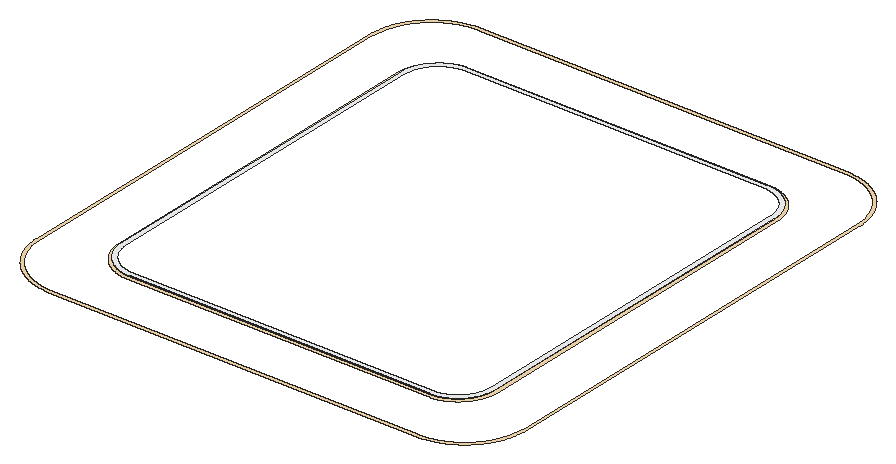
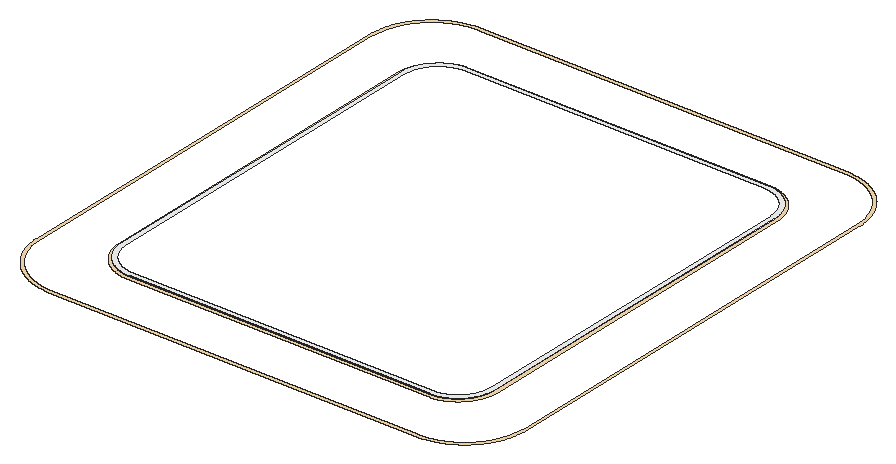
# SketchUp Ruby script. Lengths in inches.
U = 1.inch
M = Sketchup.active_model
def pt(a) = Geom::Point3d.new(a.map { |v| v * U })
def face(e, loops, mat)
  f = e.add_face(loops[0].map { |a| pt(a) })
  loops[1..].each { |l| e.add_face(l.map { |a| pt(a) }).erase! }
  f.material = f.back_material = mat if mat
  f
end
# faces: each face lists its corners as indices into pts; further lists are holes
def faces(e, pts, list, mat = nil) = list.each { |f| face(e, (f[0].is_a?(Array) ? f : [f]).map { |l| l.map { |i| pts[i] } }, mat) }
# xy, xz, yz: faces in a plane at the given z, y or x. An outline is a flat list of corners, or four numbers for a rectangle; further outlines are holes
def ring(l) = l.size == 4 ? [[l[0], l[1]], [l[2], l[1]], [l[2], l[3]], [l[0], l[3]]] : l.each_slice(2).to_a
def flat(e, list, mat, &to3) = list.each { |f| face(e, (f[0].is_a?(Array) ? f : [f]).map { |l| ring(l).map { |u, v| to3.(u, v) } }, mat) }
def xy(e, z, list, mat = nil) = flat(e, list, mat) { |x, y| [x, y, z] }
def xz(e, y, list, mat = nil) = flat(e, list, mat) { |x, z| [x, y, z] }
def yz(e, x, list, mat = nil) = flat(e, list, mat) { |y, z| [x, y, z] }
def lines(e, pts, list) = list.each { |a, b| e.add_line(pt(pts[a]), pt(pts[b])) }
# prism: a flat outline (further loops are holes) pulled along v
def prism(e, loops, v, mat = nil)
  f = face(e, loops, mat); d = Geom::Vector3d.new(v.map { |x| x * U })
  f.pushpull(f.normal.samedirection?(d) ? d.length : -d.length)
end
def box(e, o, s, mat = nil) = prism(e, [[o, [o[0] + s[0], o[1], o[2]], [o[0] + s[0], o[1] + s[1], o[2]], [o[0], o[1] + s[1], o[2]]]], [0, 0, s[2]], mat)
def at(x, y, z, deg = 0) = Geom::Transformation.translation(pt([x, y, z])) * Geom::Transformation.rotation(ORIGIN, Z_AXIS, deg.degrees)
def axes(o, x, y, z) = Geom::Transformation.new([*x, 0, *y, 0, *z, 0, *pt(o).to_a, 1])
def part(name) = M.definitions.add(name)
# library, detail: a bought-in or finely detailed component or shape, given as its bounding box
def library(name, o, s) = part(name).tap { |d| box(d.entities, o, s) }
def detail(e, o, s) = box(e.add_group.entities, o, s)
def put(e, d, t, mat = nil) = e.add_instance(d, t).tap { |i| i.material = mat if mat }
def group(e, t, mat = nil) = e.add_group.tap { |g| g.transformation = t; g.material = mat if mat }.entities
root = M.entities
M.materials.add("False Ceiling Light").color = [254, 223, 179]
M.materials.add("[Quartz Light Grey]").color = [251, 251, 252]
xy(root,115.32,[[[44.53,43.5,44.29,43.51,44.06,43.52,43.82,43.53,43.59,43.54,43.35,43.56,43.12,43.58,42.88,43.6,42.65,43.625,42.41,43.65,41.95,43.71,41.71,43.74,41.02,43.86,40.78,43.9,40.55,43.94,39.86,44.09,39.4,44.21,39.18,44.27,38.72,44.39,38.5,44.46,38.27,44.53,38.05,44.6,37.82,44.68,37.6,44.75,37.16,44.91,36.9375,44.99,36.72,45.08,36.28,45.26,36.0625,45.35,35.85,45.45,35.63,45.54,35.21,45.74,35,45.85,34.79,45.95,34.16,46.28,33.95,46.4,33.75,46.51,33.55,46.63,33.34,46.75,33.14,46.88,32.94,47,32.75,47.13,32.35,47.39,32.16,47.52,31.97,47.66,31.77,47.8,31.58,47.9375,31.4,48.08,31.21,48.22,31.02,48.37,30.84,48.51,30.48,48.81,30.3,48.97,30.12,49.12,29.94,49.28,29.77,49.4375,29.6,49.6,29.26,49.92,28.92,50.26,28.6,50.6,28.4375,50.77,28.28,50.94,28.12,51.12,27.97,51.3,27.81,51.48,27.51,51.84,27.37,52.02,27.22,52.21,27.08,52.4,26.9375,52.58,26.8,52.77,26.66,52.97,26.52,53.16,26.39,53.35,26.13,53.75,26,53.94,25.88,54.14,25.75,54.34,25.63,54.55,25.51,54.75,25.4,54.95,25.28,55.16,24.95,55.79,24.85,56,24.74,56.21,24.54,56.63,24.45,56.85,24.35,57.0625,24.26,57.28,24.08,57.72,23.99,57.9375,23.91,58.16,23.75,58.6,23.68,58.82,23.6,59.05,23.53,59.27,23.46,59.5,23.39,59.72,23.27,60.18,23.21,60.4,23.09,60.86,22.94,61.55,22.9,61.78,22.86,62.02,22.74,62.71,22.71,62.95,22.65,63.41,22.625,63.65,22.6,63.88,22.58,64.12,22.56,64.35,22.54,64.59,22.53,64.82,22.52,65.06,22.51,65.29,22.5,65.53,22.5,216.47,22.51,216.71,22.52,216.94,22.53,217.18,22.54,217.41,22.56,217.65,22.58,217.88,22.6,218.12,22.625,218.35,22.65,218.59,22.71,219.05,22.74,219.29,22.86,219.98,22.9,220.22,22.94,220.45,23.09,221.14,23.21,221.6,23.27,221.82,23.39,222.28,23.46,222.5,23.53,222.73,23.6,222.95,23.68,223.18,23.75,223.4,23.91,223.84,23.99,224.0625,24.08,224.28,24.26,224.72,24.35,224.9375,24.45,225.15,24.54,225.37,24.74,225.79,24.85,226,24.95,226.21,25.28,226.84,25.4,227.05,25.51,227.25,25.63,227.45,25.75,227.66,25.88,227.86,26,228.06,26.13,228.25,26.39,228.65,26.52,228.84,26.66,229.03,26.8,229.23,26.9375,229.42,27.08,229.6,27.22,229.79,27.37,229.98,27.51,230.16,27.81,230.52,27.97,230.7,28.12,230.88,28.28,231.06,28.4375,231.23,28.6,231.4,28.92,231.74,29.26,232.08,29.6,232.4,29.77,232.5625,29.94,232.72,30.12,232.88,30.3,233.03,30.48,233.19,30.84,233.49,31.02,233.63,31.21,233.78,31.4,233.92,31.58,234.0625,31.77,234.2,31.97,234.34,32.16,234.48,32.35,234.61,32.75,234.87,32.94,235,33.14,235.12,33.34,235.25,33.55,235.37,33.75,235.49,33.95,235.6,34.16,235.72,34.79,236.05,35,236.15,35.21,236.26,35.63,236.46,35.85,236.55,36.0625,236.65,36.28,236.74,36.72,236.92,36.9375,237.01,37.16,237.09,37.6,237.25,37.82,237.32,38.05,237.4,38.27,237.47,38.5,237.54,38.72,237.61,39.18,237.73,39.4,237.79,39.86,237.91,40.55,238.06,40.78,238.1,41.02,238.14,41.71,238.26,41.95,238.29,42.41,238.35,42.65,238.375,42.88,238.4,43.12,238.42,43.35,238.44,43.59,238.46,43.82,238.47,44.06,238.48,44.29,238.49,44.53,238.5,177.47,238.5,177.71,238.49,177.94,238.48,178.18,238.47,178.41,238.46,178.65,238.44,178.88,238.42,179.12,238.4,179.35,238.375,179.59,238.35,180.05,238.29,180.29,238.26,180.98,238.14,181.22,238.1,181.45,238.06,182.14,237.91,182.6,237.79,182.82,237.73,183.28,237.61,183.5,237.54,183.73,237.47,183.95,237.4,184.18,237.32,184.4,237.25,184.84,237.09,185.0625,237.01,185.28,236.92,185.72,236.74,185.9375,236.65,186.15,236.55,186.37,236.46,186.79,236.26,187,236.15,187.21,236.05,187.84,235.72,188.05,235.6,188.25,235.49,188.45,235.37,188.66,235.25,188.86,235.12,189.06,235,189.25,234.87,189.65,234.61,189.84,234.48,190.03,234.34,190.23,234.2,190.42,234.0625,190.6,233.92,190.79,233.78,190.98,233.63,191.16,233.49,191.52,233.19,191.7,233.03,191.88,232.88,192.06,232.72,192.23,232.5625,192.4,232.4,192.74,232.08,193.08,231.74,193.4,231.4,193.5625,231.23,193.72,231.06,193.88,230.88,194.03,230.7,194.19,230.52,194.49,230.16,194.63,229.98,194.78,229.79,194.92,229.6,195.0625,229.42,195.2,229.23,195.34,229.03,195.48,228.84,195.61,228.65,195.87,228.25,196,228.06,196.12,227.86,196.25,227.66,196.37,227.45,196.49,227.25,196.6,227.05,196.72,226.84,197.05,226.21,197.15,226,197.26,225.79,197.46,225.37,197.55,225.15,197.65,224.9375,197.74,224.72,197.92,224.28,198.01,224.0625,198.09,223.84,198.25,223.4,198.32,223.18,198.4,222.95,198.47,222.73,198.54,222.5,198.61,222.28,198.73,221.82,198.79,221.6,198.91,221.14,199.06,220.45,199.1,220.22,199.14,219.98,199.26,219.29,199.29,219.05,199.35,218.59,199.375,218.35,199.4,218.12,199.42,217.88,199.44,217.65,199.46,217.41,199.47,217.18,199.48,216.94,199.49,216.71,199.5,216.47,199.5,65.53,199.49,65.29,199.48,65.06,199.47,64.82,199.46,64.59,199.44,64.35,199.42,64.12,199.4,63.88,199.375,63.65,199.35,63.41,199.29,62.95,199.26,62.71,199.14,62.02,199.1,61.78,199.06,61.55,198.91,60.86,198.79,60.4,198.73,60.18,198.61,59.72,198.54,59.5,198.47,59.27,198.4,59.05,198.32,58.82,198.25,58.6,198.09,58.16,198.01,57.9375,197.92,57.72,197.74,57.28,197.65,57.0625,197.55,56.85,197.46,56.63,197.26,56.21,197.15,56,197.05,55.79,196.72,55.16,196.6,54.95,196.49,54.75,196.37,54.55,196.25,54.34,196.12,54.14,196,53.94,195.87,53.75,195.61,53.35,195.48,53.16,195.34,52.97,195.2,52.77,195.0625,52.58,194.92,52.4,194.78,52.21,194.63,52.02,194.49,51.84,194.19,51.48,194.03,51.3,193.88,51.12,193.72,50.94,193.5625,50.77,193.4,50.6,193.08,50.26,192.74,49.92,192.4,49.6,192.23,49.4375,192.06,49.28,191.88,49.12,191.7,48.97,191.52,48.81,191.16,48.51,190.98,48.37,190.79,48.22,190.6,48.08,190.42,47.9375,190.23,47.8,190.03,47.66,189.84,47.52,189.65,47.39,189.25,47.13,189.06,47,188.86,46.88,188.66,46.75,188.45,46.63,188.25,46.51,188.05,46.4,187.84,46.28,187.21,45.95,187,45.85,186.79,45.74,186.37,45.54,186.15,45.45,185.9375,45.35,185.72,45.26,185.28,45.08,185.0625,44.99,184.84,44.91,184.4,44.75,184.18,44.68,183.95,44.6,183.73,44.53,183.5,44.46,183.28,44.39,182.82,44.27,182.6,44.21,182.14,44.09,181.45,43.94,181.22,43.9,180.98,43.86,180.29,43.74,180.05,43.71,179.59,43.65,179.35,43.625,179.12,43.6,178.88,43.58,178.65,43.56,178.41,43.54,178.18,43.53,177.94,43.52,177.71,43.51,177.47,43.5],[44.55,44.5,177.45,44.5,177.68,44.51,177.9,44.52,178.35,44.54,178.57,44.56,178.8,44.58,179.02,44.6,179.25,44.62,179.47,44.64,179.69,44.67,179.92,44.7,180.36,44.76,180.59,44.8,181.25,44.92,182.13,45.12,182.35,45.18,182.56,45.23,183,45.35,183.21,45.42,183.43,45.48,183.64,45.55,183.86,45.625,184.07,45.7,184.28,45.77,184.91,46.01,185.125,46.09,185.33,46.18,185.54,46.27,185.74,46.36,185.95,46.45,186.15,46.55,186.36,46.64,186.76,46.84,186.96,46.95,187.16,47.05,187.36,47.16,187.55,47.27,187.75,47.38,187.94,47.49,188.14,47.61,188.9,48.09,189.08,48.22,189.27,48.35,189.45,48.47,189.64,48.61,189.82,48.74,190.18,49.01,190.35,49.15,190.53,49.29,190.7,49.43,190.88,49.58,191.05,49.72,191.39,50.02,191.55,50.17,191.72,50.33,191.88,50.48,192.52,51.12,192.67,51.28,192.83,51.45,192.98,51.61,193.28,51.95,193.42,52.12,193.57,52.3,193.71,52.47,193.85,52.65,193.99,52.82,194.26,53.18,194.39,53.36,194.53,53.55,194.65,53.73,194.78,53.92,194.91,54.1,195.39,54.86,195.51,55.06,195.62,55.25,195.73,55.45,195.84,55.64,195.95,55.84,196.05,56.04,196.16,56.24,196.36,56.64,196.45,56.85,196.55,57.05,196.64,57.26,196.73,57.46,196.82,57.67,196.91,57.875,196.99,58.09,197.23,58.72,197.3,58.93,197.375,59.14,197.45,59.36,197.52,59.57,197.58,59.79,197.65,60,197.77,60.44,197.82,60.65,197.88,60.87,198.08,61.75,198.2,62.41,198.24,62.64,198.3,63.08,198.33,63.31,198.36,63.53,198.38,63.75,198.4,63.98,198.42,64.2,198.44,64.43,198.46,64.65,198.48,65.1,198.49,65.32,198.5,65.55,198.5,216.45,198.49,216.68,198.48,216.9,198.46,217.35,198.44,217.57,198.42,217.8,198.4,218.02,198.38,218.25,198.36,218.47,198.33,218.69,198.3,218.92,198.24,219.36,198.2,219.59,198.08,220.25,197.88,221.13,197.82,221.35,197.77,221.56,197.65,222,197.58,222.21,197.52,222.43,197.45,222.64,197.375,222.86,197.3,223.07,197.23,223.28,196.99,223.91,196.91,224.125,196.82,224.33,196.73,224.54,196.64,224.74,196.55,224.95,196.45,225.15,196.36,225.36,196.16,225.76,196.05,225.96,195.95,226.16,195.84,226.36,195.73,226.55,195.62,226.75,195.51,226.94,195.39,227.14,194.91,227.9,194.78,228.08,194.65,228.27,194.53,228.45,194.39,228.64,194.26,228.82,193.99,229.18,193.85,229.35,193.71,229.53,193.57,229.7,193.42,229.88,193.28,230.05,192.98,230.39,192.83,230.55,192.67,230.72,192.52,230.88,191.88,231.52,191.72,231.67,191.55,231.83,191.39,231.98,191.05,232.28,190.88,232.42,190.7,232.57,190.53,232.71,190.35,232.85,190.18,232.99,189.82,233.26,189.64,233.39,189.45,233.53,189.27,233.65,189.08,233.78,188.9,233.91,188.14,234.39,187.94,234.51,187.75,234.62,187.55,234.73,187.36,234.84,187.16,234.95,186.96,235.05,186.76,235.16,186.36,235.36,186.15,235.45,185.95,235.55,185.74,235.64,185.54,235.73,185.33,235.82,185.125,235.91,184.91,235.99,184.28,236.23,184.07,236.3,183.86,236.375,183.64,236.45,183.43,236.52,183.21,236.58,183,236.65,182.56,236.77,182.35,236.82,182.13,236.88,181.25,237.08,180.59,237.2,180.36,237.24,179.92,237.3,179.69,237.33,179.47,237.36,179.25,237.38,179.02,237.4,178.8,237.42,178.57,237.44,178.35,237.46,177.9,237.48,177.68,237.49,177.45,237.5,44.55,237.5,44.32,237.49,44.1,237.48,43.65,237.46,43.43,237.44,43.2,237.42,42.98,237.4,42.75,237.38,42.53,237.36,42.31,237.33,42.08,237.3,41.64,237.24,41.41,237.2,40.75,237.08,39.87,236.88,39.65,236.82,39.44,236.77,39,236.65,38.79,236.58,38.57,236.52,38.36,236.45,38.14,236.375,37.93,236.3,37.72,236.23,37.09,235.99,36.875,235.91,36.67,235.82,36.46,235.73,36.26,235.64,36.05,235.55,35.85,235.45,35.64,235.36,35.24,235.16,35.04,235.05,34.84,234.95,34.64,234.84,34.45,234.73,34.25,234.62,34.06,234.51,33.86,234.39,33.1,233.91,32.92,233.78,32.73,233.65,32.55,233.53,32.36,233.39,32.18,233.26,31.82,232.99,31.65,232.85,31.47,232.71,31.3,232.57,31.12,232.42,30.95,232.28,30.61,231.98,30.45,231.83,30.28,231.67,30.12,231.52,29.48,230.88,29.33,230.72,29.17,230.55,29.02,230.39,28.72,230.05,28.58,229.88,28.43,229.7,28.29,229.53,28.15,229.35,28.01,229.18,27.74,228.82,27.61,228.64,27.47,228.45,27.35,228.27,27.22,228.08,27.09,227.9,26.61,227.14,26.49,226.94,26.38,226.75,26.27,226.55,26.16,226.36,26.05,226.16,25.95,225.96,25.84,225.76,25.64,225.36,25.55,225.15,25.45,224.95,25.36,224.74,25.27,224.54,25.18,224.33,25.09,224.125,25.01,223.91,24.77,223.28,24.7,223.07,24.625,222.86,24.55,222.64,24.48,222.43,24.42,222.21,24.35,222,24.23,221.56,24.18,221.35,24.12,221.13,23.92,220.25,23.8,219.59,23.76,219.36,23.7,218.92,23.67,218.69,23.64,218.47,23.62,218.25,23.6,218.02,23.58,217.8,23.56,217.57,23.54,217.35,23.52,216.9,23.51,216.68,23.5,216.45,23.5,65.55,23.51,65.32,23.52,65.1,23.54,64.65,23.56,64.43,23.58,64.2,23.6,63.98,23.62,63.75,23.64,63.53,23.67,63.31,23.7,63.08,23.76,62.64,23.8,62.41,23.92,61.75,24.12,60.87,24.18,60.65,24.23,60.44,24.35,60,24.42,59.79,24.48,59.57,24.55,59.36,24.625,59.14,24.7,58.93,24.77,58.72,25.01,58.09,25.09,57.875,25.18,57.67,25.27,57.46,25.36,57.26,25.45,57.05,25.55,56.85,25.64,56.64,25.84,56.24,25.95,56.04,26.05,55.84,26.16,55.64,26.27,55.45,26.38,55.25,26.49,55.06,26.61,54.86,27.09,54.1,27.22,53.92,27.35,53.73,27.47,53.55,27.61,53.36,27.74,53.18,28.01,52.82,28.15,52.65,28.29,52.47,28.43,52.3,28.58,52.12,28.72,51.95,29.02,51.61,29.17,51.45,29.33,51.28,29.48,51.12,30.12,50.48,30.28,50.33,30.45,50.17,30.61,50.02,30.95,49.72,31.12,49.58,31.3,49.43,31.47,49.29,31.65,49.15,31.82,49.01,32.18,48.74,32.36,48.61,32.55,48.47,32.73,48.35,32.92,48.22,33.1,48.09,33.86,47.61,34.06,47.49,34.25,47.38,34.45,47.27,34.64,47.16,34.84,47.05,35.04,46.95,35.24,46.84,35.64,46.64,35.85,46.55,36.05,46.45,36.26,46.36,36.46,46.27,36.67,46.18,36.875,46.09,37.09,46.01,37.72,45.77,37.93,45.7,38.14,45.625,38.36,45.55,38.57,45.48,38.79,45.42,39,45.35,39.44,45.23,39.65,45.18,39.87,45.12,40.75,44.92,41.41,44.8,41.64,44.76,42.08,44.7,42.31,44.67,42.53,44.64,42.75,44.62,42.98,44.6,43.2,44.58,43.43,44.56,43.65,44.54,44.1,44.52,44.32,44.51]],[[56.62,63.5,55.86,63.54,55.67,63.5625,55.48,63.58,55.29,63.6,54.91,63.65,54.72,63.68,54.54,63.71,54.35,63.74,54.16,63.78,53.98,63.82,53.6,63.9,53.42,63.95,53.23,64,52.87,64.1,52.6875,64.16,52.5,64.21,52.32,64.27,52.14,64.34,51.97,64.4,51.43,64.61,51.26,64.69,51.08,64.76,50.74,64.92,50.57,65.01,50.4,65.09,49.89,65.36,49.73,65.46,49.5625,65.55,49.4,65.65,49.08,65.85,48.76,66.07,48.61,66.18,48.45,66.29,48.3,66.4,48.15,66.52,48,66.63,47.85,66.75,47.7,66.875,47.56,67,47.41,67.12,47.27,67.25,47.13,67.375,46.99,67.51,46.86,67.64,46.72,67.77,46.46,68.05,46.33,68.1875,46.2,68.33,46.07,68.47,45.95,68.61,45.82,68.76,45.7,68.91,45.59,69.06,45.35,69.36,45.24,69.51,45.02,69.83,44.92,69.98,44.8125,70.14,44.71,70.3,44.61,70.47,44.51,70.63,44.42,70.79,44.32,70.96,44.23,71.125,44.14,71.3,43.97,71.64,43.73,72.15,43.66,72.33,43.58,72.5,43.44,72.86,43.375,73.04,43.25,73.4,43.13,73.76,43.08,73.94,42.98,74.31,42.93,74.49,42.89,74.68,42.84,74.86,42.8,75.05,42.77,75.24,42.73,75.42,42.61,76.18,42.59,76.37,42.57,76.55,42.55,76.74,42.54,76.93,42.53,77.125,42.51,77.5,42.5,77.7,42.5,204.38,42.54,205.14,42.5625,205.33,42.58,205.52,42.6,205.7,42.65,206.08,42.71,206.46,42.74,206.64,42.78,206.83,42.82,207.01,42.86,207.2,42.9,207.38,42.95,207.57,42.99,207.75,43.04,207.9375,43.1,208.12,43.15,208.3,43.33,208.84,43.4,209.02,43.46,209.2,43.6,209.55,43.68,209.72,43.75,209.9,43.91,210.24,44,210.41,44.08,210.58,44.35,211.09,44.44,211.25,44.54,211.41,44.64,211.58,44.94,212.06,45.05,212.21,45.16,212.37,45.27,212.52,45.38,212.68,45.5,212.83,45.61,212.98,45.85,213.27,45.97,213.42,46.1,213.5625,46.22,213.7,46.61,214.12,46.75,214.25,46.88,214.39,47.3,214.78,47.4375,214.9,47.58,215.03,47.73,215.15,48.02,215.39,48.17,215.5,48.32,215.62,48.48,215.73,48.63,215.84,48.79,215.95,48.94,216.06,49.42,216.36,49.59,216.46,49.75,216.56,49.91,216.65,50.42,216.92,50.59,217,50.76,217.09,51.1,217.25,51.28,217.32,51.45,217.4,51.8,217.54,51.98,217.6,52.16,217.67,52.7,217.85,52.88,217.9,53.0625,217.96,53.25,218.01,53.43,218.05,53.62,218.1,53.8,218.14,53.99,218.18,54.17,218.22,54.36,218.26,54.54,218.29,54.92,218.35,55.3,218.4,55.48,218.42,55.67,218.4375,55.86,218.46,56.62,218.5,165.38,218.5,166.14,218.46,166.33,218.4375,166.52,218.42,166.7,218.4,167.08,218.35,167.46,218.29,167.64,218.26,167.83,218.22,168.01,218.18,168.2,218.14,168.38,218.1,168.57,218.05,168.75,218.01,168.9375,217.96,169.12,217.9,169.3,217.85,169.84,217.67,170.02,217.6,170.2,217.54,170.55,217.4,170.72,217.32,170.9,217.25,171.24,217.09,171.41,217,171.58,216.92,172.09,216.65,172.25,216.56,172.41,216.46,172.58,216.36,173.06,216.06,173.21,215.95,173.37,215.84,173.52,215.73,173.68,215.62,173.83,215.5,173.98,215.39,174.27,215.15,174.42,215.03,174.5625,214.9,174.7,214.78,175.12,214.39,175.25,214.25,175.39,214.12,175.78,213.7,175.9,213.5625,176.03,213.42,176.15,213.27,176.39,212.98,176.5,212.83,176.62,212.68,176.73,212.52,176.84,212.37,176.95,212.21,177.06,212.06,177.36,211.58,177.46,211.41,177.56,211.25,177.65,211.09,177.92,210.58,178,210.41,178.09,210.24,178.25,209.9,178.32,209.72,178.4,209.55,178.54,209.2,178.6,209.02,178.67,208.84,178.85,208.3,178.9,208.12,178.96,207.9375,179.01,207.75,179.05,207.57,179.1,207.38,179.14,207.2,179.18,207.01,179.22,206.83,179.26,206.64,179.29,206.46,179.35,206.08,179.4,205.7,179.42,205.52,179.4375,205.33,179.46,205.14,179.5,204.38,179.5,77.62,179.46,76.86,179.4375,76.67,179.42,76.48,179.4,76.3,179.35,75.92,179.29,75.54,179.26,75.36,179.22,75.17,179.18,74.99,179.14,74.8,179.1,74.62,179.05,74.43,179.01,74.25,178.96,74.0625,178.9,73.88,178.85,73.7,178.67,73.16,178.6,72.98,178.54,72.8,178.4,72.45,178.32,72.28,178.25,72.1,178.09,71.76,178,71.59,177.92,71.42,177.65,70.91,177.56,70.75,177.46,70.59,177.36,70.42,177.06,69.94,176.95,69.79,176.84,69.63,176.73,69.48,176.62,69.32,176.5,69.17,176.39,69.02,176.15,68.73,176.03,68.58,175.9,68.4375,175.78,68.3,175.39,67.88,175.25,67.75,175.12,67.61,174.7,67.22,174.5625,67.1,174.42,66.97,174.27,66.85,173.98,66.61,173.83,66.5,173.68,66.38,173.52,66.27,173.37,66.16,173.21,66.05,173.06,65.94,172.58,65.64,172.41,65.54,172.25,65.44,172.09,65.35,171.58,65.08,171.41,65,171.24,64.91,170.9,64.75,170.72,64.68,170.55,64.6,170.2,64.46,170.02,64.4,169.84,64.33,169.3,64.15,169.12,64.1,168.9375,64.04,168.75,63.99,168.57,63.95,168.38,63.9,168.2,63.86,168.01,63.82,167.83,63.78,167.64,63.74,167.46,63.71,167.08,63.65,166.7,63.6,166.52,63.58,166.33,63.5625,166.14,63.54,165.38,63.5],[56.65,64.5,165.35,64.5,165.71,64.52,165.88,64.53,166.06,64.54,166.24,64.56,166.41,64.57,166.59,64.59,166.76,64.62,166.9375,64.64,167.11,64.67,167.29,64.69,167.46,64.73,167.63,64.76,167.81,64.79,168.15,64.87,168.32,64.92,168.49,64.96,169.17,65.16,169.34,65.22,169.51,65.27,169.67,65.33,169.84,65.4,170,65.46,170.17,65.53,170.65,65.74,170.8125,65.82,170.97,65.89,171.29,66.05,171.44,66.14,171.6,66.22,172.2,66.58,172.5,66.78,172.65,66.875,172.79,66.98,172.94,67.08,173.08,67.18,173.5,67.51,173.63,67.62,173.77,67.73,174.55,68.45,175.27,69.23,175.38,69.37,175.49,69.5,175.82,69.92,175.92,70.06,176.02,70.21,176.125,70.35,176.22,70.5,176.42,70.8,176.78,71.4,176.86,71.56,176.95,71.71,177.11,72.03,177.18,72.1875,177.26,72.35,177.47,72.83,177.54,73,177.6,73.16,177.67,73.33,177.73,73.49,177.78,73.66,177.84,73.83,178.04,74.51,178.08,74.68,178.13,74.85,178.21,75.19,178.24,75.37,178.27,75.54,178.31,75.71,178.33,75.89,178.36,76.0625,178.38,76.24,178.41,76.41,178.43,76.59,178.44,76.76,178.46,76.94,178.47,77.12,178.48,77.29,178.5,77.65,178.5,204.35,178.48,204.71,178.47,204.88,178.46,205.06,178.44,205.24,178.43,205.41,178.41,205.59,178.38,205.76,178.36,205.9375,178.33,206.11,178.31,206.29,178.27,206.46,178.24,206.63,178.21,206.81,178.13,207.15,178.08,207.32,178.04,207.49,177.84,208.17,177.78,208.34,177.73,208.51,177.67,208.67,177.6,208.84,177.54,209,177.47,209.17,177.26,209.65,177.18,209.8125,177.11,209.97,176.95,210.29,176.86,210.44,176.78,210.6,176.42,211.2,176.22,211.5,176.125,211.65,176.02,211.79,175.92,211.94,175.82,212.08,175.49,212.5,175.38,212.63,175.27,212.77,174.55,213.55,173.77,214.27,173.63,214.38,173.5,214.49,173.08,214.82,172.94,214.92,172.79,215.02,172.65,215.125,172.5,215.22,172.2,215.42,171.6,215.78,171.44,215.86,171.29,215.95,170.97,216.11,170.8125,216.18,170.65,216.26,170.17,216.47,170,216.54,169.84,216.6,169.67,216.67,169.51,216.73,169.34,216.78,169.17,216.84,168.49,217.04,168.32,217.08,168.15,217.13,167.81,217.21,167.63,217.24,167.46,217.27,167.29,217.31,167.11,217.33,166.9375,217.36,166.76,217.38,166.59,217.41,166.41,217.43,166.24,217.44,166.06,217.46,165.88,217.47,165.71,217.48,165.35,217.5,56.65,217.5,56.29,217.48,56.12,217.47,55.94,217.46,55.76,217.44,55.59,217.43,55.41,217.41,55.24,217.38,55.0625,217.36,54.89,217.33,54.71,217.31,54.54,217.27,54.37,217.24,54.19,217.21,53.85,217.13,53.68,217.08,53.51,217.04,52.83,216.84,52.66,216.78,52.49,216.73,52.33,216.67,52.16,216.6,52,216.54,51.83,216.47,51.35,216.26,51.1875,216.18,51.03,216.11,50.71,215.95,50.56,215.86,50.4,215.78,49.8,215.42,49.5,215.22,49.35,215.125,49.21,215.02,49.06,214.92,48.92,214.82,48.5,214.49,48.37,214.38,48.23,214.27,47.45,213.55,46.73,212.77,46.62,212.63,46.51,212.5,46.18,212.08,46.08,211.94,45.98,211.79,45.875,211.65,45.78,211.5,45.58,211.2,45.22,210.6,45.14,210.44,45.05,210.29,44.89,209.97,44.82,209.8125,44.74,209.65,44.53,209.17,44.46,209,44.4,208.84,44.33,208.67,44.27,208.51,44.22,208.34,44.16,208.17,43.96,207.49,43.92,207.32,43.87,207.15,43.79,206.81,43.76,206.63,43.73,206.46,43.69,206.29,43.67,206.11,43.64,205.9375,43.62,205.76,43.59,205.59,43.57,205.41,43.56,205.24,43.54,205.06,43.53,204.88,43.52,204.71,43.5,204.35,43.5,77.72,43.51,77.54,43.51,77.36,43.52,77.18,43.54,77.01,43.55,76.83,43.57,76.65,43.59,76.48,43.61,76.3,43.63,76.125,43.66,75.95,43.68,75.78,43.71,75.6,43.75,75.43,43.78,75.25,43.86,74.91,43.9,74.73,43.94,74.5625,43.99,74.39,44.14,73.88,44.2,73.71,44.26,73.55,44.38,73.21,44.44,73.05,44.51,72.88,44.65,72.56,44.72,72.39,44.79,72.23,44.87,72.07,44.95,71.92,45.11,71.6,45.2,71.45,45.29,71.29,45.375,71.14,45.47,70.99,45.56,70.83,45.65,70.68,45.75,70.54,45.95,70.24,46.05,70.1,46.16,69.96,46.26,69.8125,46.375,69.67,46.48,69.54,46.6,69.4,46.71,69.26,46.82,69.13,46.94,68.99,47.0625,68.86,47.18,68.73,47.43,68.48,47.55,68.35,47.68,68.23,47.8125,68.11,47.94,67.99,48.07,67.87,48.21,67.76,48.34,67.64,49.04,67.09,49.1875,66.99,49.33,66.89,49.48,66.79,49.625,66.69,49.77,66.6,49.93,66.5,50.38,66.23,50.54,66.15,50.69,66.0625,50.85,65.98,51.17,65.82,51.33,65.75,51.49,65.67,51.65,65.6,51.82,65.53,51.98,65.47,52.15,65.4,52.3125,65.34,52.48,65.28,52.65,65.22,52.81,65.17,52.98,65.11,53.49,64.96,53.67,64.92,53.84,64.875,54.01,64.84,54.18,64.8,54.36,64.76,54.53,64.73,54.71,64.7,54.88,64.67,55.06,64.64,55.23,64.62,55.41,64.59,55.58,64.57,55.76,64.56,55.9375,64.54,56.11,64.53]]],"False Ceiling Light")
xy(root,115.91,[[[56.65,64.5,165.35,64.5,165.71,64.52,165.88,64.53,166.06,64.54,166.24,64.56,166.41,64.57,166.59,64.59,166.76,64.62,166.9375,64.64,167.11,64.67,167.29,64.69,167.46,64.73,167.63,64.76,167.81,64.79,168.15,64.87,168.32,64.92,168.49,64.96,169.17,65.16,169.34,65.22,169.51,65.27,169.67,65.33,169.84,65.4,170,65.46,170.17,65.53,170.65,65.74,170.8125,65.82,170.97,65.89,171.29,66.05,171.44,66.14,171.6,66.22,172.2,66.58,172.5,66.78,172.65,66.875,172.79,66.98,172.94,67.08,173.08,67.18,173.5,67.51,173.63,67.62,173.77,67.73,174.55,68.45,175.27,69.23,175.38,69.37,175.49,69.5,175.82,69.92,175.92,70.06,176.02,70.21,176.125,70.35,176.22,70.5,176.42,70.8,176.78,71.4,176.86,71.56,176.95,71.71,177.11,72.03,177.18,72.1875,177.26,72.35,177.47,72.83,177.54,73,177.6,73.16,177.67,73.33,177.73,73.49,177.78,73.66,177.84,73.83,178.04,74.51,178.08,74.68,178.13,74.85,178.21,75.19,178.24,75.37,178.27,75.54,178.31,75.71,178.33,75.89,178.36,76.0625,178.38,76.24,178.41,76.41,178.43,76.59,178.44,76.76,178.46,76.94,178.47,77.12,178.48,77.29,178.5,77.65,178.5,204.35,178.48,204.71,178.47,204.88,178.46,205.06,178.44,205.24,178.43,205.41,178.41,205.59,178.38,205.76,178.36,205.9375,178.33,206.11,178.31,206.29,178.27,206.46,178.24,206.63,178.21,206.81,178.13,207.15,178.08,207.32,178.04,207.49,177.84,208.17,177.78,208.34,177.73,208.51,177.67,208.67,177.6,208.84,177.54,209,177.47,209.17,177.26,209.65,177.18,209.8125,177.11,209.97,176.95,210.29,176.86,210.44,176.78,210.6,176.42,211.2,176.22,211.5,176.125,211.65,176.02,211.79,175.92,211.94,175.82,212.08,175.49,212.5,175.38,212.63,175.27,212.77,174.55,213.55,173.77,214.27,173.63,214.38,173.5,214.49,173.08,214.82,172.94,214.92,172.79,215.02,172.65,215.125,172.5,215.22,172.2,215.42,171.6,215.78,171.44,215.86,171.29,215.95,170.97,216.11,170.8125,216.18,170.65,216.26,170.17,216.47,170,216.54,169.84,216.6,169.67,216.67,169.51,216.73,169.34,216.78,169.17,216.84,168.49,217.04,168.32,217.08,168.15,217.13,167.81,217.21,167.63,217.24,167.46,217.27,167.29,217.31,167.11,217.33,166.9375,217.36,166.76,217.38,166.59,217.41,166.41,217.43,166.24,217.44,166.06,217.46,165.88,217.47,165.71,217.48,165.35,217.5,56.65,217.5,56.29,217.48,56.12,217.47,55.94,217.46,55.76,217.44,55.59,217.43,55.41,217.41,55.24,217.38,55.0625,217.36,54.89,217.33,54.71,217.31,54.54,217.27,54.37,217.24,54.19,217.21,53.85,217.13,53.68,217.08,53.51,217.04,52.83,216.84,52.66,216.78,52.49,216.73,52.33,216.67,52.16,216.6,52,216.54,51.83,216.47,51.35,216.26,51.1875,216.18,51.03,216.11,50.71,215.95,50.56,215.86,50.4,215.78,49.8,215.42,49.5,215.22,49.35,215.125,49.21,215.02,49.06,214.92,48.92,214.82,48.5,214.49,48.37,214.38,48.23,214.27,47.45,213.55,46.73,212.77,46.62,212.63,46.51,212.5,46.18,212.08,46.08,211.94,45.98,211.79,45.875,211.65,45.78,211.5,45.58,211.2,45.22,210.6,45.14,210.44,45.05,210.29,44.89,209.97,44.82,209.8125,44.74,209.65,44.53,209.17,44.46,209,44.4,208.84,44.33,208.67,44.27,208.51,44.22,208.34,44.16,208.17,43.96,207.49,43.92,207.32,43.87,207.15,43.79,206.81,43.76,206.63,43.73,206.46,43.69,206.29,43.67,206.11,43.64,205.9375,43.62,205.76,43.59,205.59,43.57,205.41,43.56,205.24,43.54,205.06,43.53,204.88,43.52,204.71,43.5,204.35,43.5,77.72,43.51,77.54,43.51,77.36,43.52,77.18,43.54,77.01,43.55,76.83,43.57,76.65,43.59,76.48,43.61,76.3,43.63,76.125,43.66,75.95,43.68,75.78,43.71,75.6,43.75,75.43,43.78,75.25,43.86,74.91,43.9,74.73,43.94,74.5625,43.99,74.39,44.14,73.88,44.2,73.71,44.26,73.55,44.38,73.21,44.44,73.05,44.51,72.88,44.65,72.56,44.72,72.39,44.79,72.23,44.87,72.07,44.95,71.92,45.11,71.6,45.2,71.45,45.29,71.29,45.375,71.14,45.47,70.99,45.56,70.83,45.65,70.68,45.75,70.54,45.95,70.24,46.05,70.1,46.16,69.96,46.26,69.8125,46.375,69.67,46.48,69.54,46.6,69.4,46.71,69.26,46.82,69.13,46.94,68.99,47.0625,68.86,47.18,68.73,47.43,68.48,47.55,68.35,47.68,68.23,47.8125,68.11,47.94,67.99,48.07,67.87,48.21,67.76,48.34,67.64,49.04,67.09,49.1875,66.99,49.33,66.89,49.48,66.79,49.625,66.69,49.77,66.6,49.93,66.5,50.38,66.23,50.54,66.15,50.69,66.0625,50.85,65.98,51.17,65.82,51.33,65.75,51.49,65.67,51.65,65.6,51.82,65.53,51.98,65.47,52.15,65.4,52.3125,65.34,52.48,65.28,52.65,65.22,52.81,65.17,52.98,65.11,53.49,64.96,53.67,64.92,53.84,64.875,54.01,64.84,54.18,64.8,54.36,64.76,54.53,64.73,54.71,64.7,54.88,64.67,55.06,64.64,55.23,64.62,55.41,64.59,55.58,64.57,55.76,64.56,55.9375,64.54,56.11,64.53],[56.68,66,56.53,66.01,56.21,66.03,56.06,66.04,55.9,66.05,55.74,66.07,55.58,66.08,55.43,66.1,55.27,66.125,55.12,66.15,54.96,66.17,54.81,66.2,54.65,66.23,54.5,66.26,54.34,66.3,54.1875,66.33,54.04,66.37,53.88,66.41,53.73,66.45,53.58,66.5,53.43,66.54,52.98,66.69,52.83,66.75,52.6875,66.8,52.54,66.86,52.39,66.92,52.25,66.98,52.1,67.04,51.26,67.46,50.98,67.62,50.85,67.7,50.71,67.78,50.58,67.86,50.44,67.95,50.3125,68.04,50.18,68.125,50.05,68.21,49.93,68.31,49.8,68.4,49.67,68.5,49.55,68.59,49.19,68.89,49.07,69,48.95,69.1,48.83,69.21,48.72,69.32,48.6,69.43,48.27,69.76,48.17,69.88,48.06,70,47.96,70.11,47.85,70.23,47.75,70.35,47.65,70.48,47.55,70.6,47.46,70.72,47.36,70.85,46.91,71.5,46.75,71.76,46.59,72.04,46.51,72.17,46.43,72.3125,46.36,72.45,46.22,72.73,46.08,73.02,46.02,73.16,45.96,73.31,45.9,73.45,45.84,73.6,45.78,73.74,45.72,73.89,45.52,74.49,45.48,74.64,45.4375,74.79,45.36,75.1,45.28,75.4,45.25,75.56,45.22,75.71,45.19,75.87,45.16,76.02,45.14,76.18,45.12,76.33,45.08,76.65,45.06,76.8,45.04,76.96,45.02,77.28,45.01,77.43,45.01,77.59,45,77.75,45,204.3125,45.01,204.47,45.02,204.63,45.03,204.78,45.05,205.1,45.07,205.25,45.08,205.41,45.1,205.57,45.125,205.72,45.15,205.88,45.17,206.03,45.2,206.1875,45.23,206.34,45.26,206.49,45.3,206.65,45.33,206.8,45.37,206.95,45.41,207.11,45.49,207.41,45.64,207.86,45.6875,208.01,45.74,208.15,45.8,208.3,45.85,208.45,45.91,208.59,45.97,208.74,46.04,208.88,46.1,209.02,46.17,209.17,46.45,209.73,46.53,209.86,46.61,210,46.6875,210.14,46.77,210.27,46.85,210.4,46.9375,210.54,47.02,210.67,47.2,210.93,47.29,211.05,47.38,211.18,47.48,211.31,47.58,211.43,47.67,211.55,47.77,211.67,47.98,211.91,48.08,212.03,48.1875,212.15,48.3,212.26,48.4,212.375,48.51,212.49,48.625,212.6,48.74,212.7,48.85,212.8125,48.97,212.92,49.09,213.02,49.33,213.23,49.45,213.33,49.57,213.42,49.69,213.52,49.82,213.62,49.95,213.71,50.07,213.8,50.33,213.98,50.46,214.0625,50.6,214.15,50.73,214.23,50.86,214.3125,51,214.39,51.14,214.47,51.27,214.55,51.83,214.83,51.98,214.9,52.12,214.96,52.26,215.03,52.41,215.09,52.55,215.15,52.7,215.2,52.85,215.26,52.99,215.3125,53.14,215.36,53.59,215.51,53.89,215.59,54.05,215.63,54.2,215.67,54.35,215.7,54.51,215.74,54.66,215.77,54.8125,215.8,54.97,215.83,55.12,215.85,55.28,215.875,55.43,215.9,55.59,215.92,55.75,215.93,55.9,215.95,56.22,215.97,56.37,215.98,56.53,215.99,56.6875,216,165.3125,216,165.47,215.99,165.63,215.98,165.78,215.97,166.1,215.95,166.25,215.93,166.41,215.92,166.57,215.9,166.72,215.875,166.88,215.85,167.03,215.83,167.1875,215.8,167.34,215.77,167.49,215.74,167.65,215.7,167.8,215.67,167.95,215.63,168.11,215.59,168.41,215.51,168.86,215.36,169.01,215.3125,169.15,215.26,169.3,215.2,169.45,215.15,169.59,215.09,169.74,215.03,169.88,214.96,170.02,214.9,170.17,214.83,170.73,214.55,170.86,214.47,171,214.39,171.14,214.3125,171.27,214.23,171.4,214.15,171.54,214.0625,171.67,213.98,171.93,213.8,172.05,213.71,172.18,213.62,172.31,213.52,172.43,213.42,172.55,213.33,172.67,213.23,172.91,213.02,173.03,212.92,173.15,212.8125,173.26,212.7,173.375,212.6,173.49,212.49,173.6,212.375,173.7,212.26,173.8125,212.15,173.92,212.03,174.02,211.91,174.23,211.67,174.33,211.55,174.42,211.43,174.52,211.31,174.62,211.18,174.71,211.05,174.8,210.93,174.98,210.67,175.0625,210.54,175.15,210.4,175.23,210.27,175.3125,210.14,175.39,210,175.47,209.86,175.55,209.73,175.83,209.17,175.9,209.02,175.96,208.88,176.03,208.74,176.09,208.59,176.15,208.45,176.2,208.3,176.26,208.15,176.3125,208.01,176.36,207.86,176.51,207.41,176.59,207.11,176.63,206.95,176.67,206.8,176.7,206.65,176.74,206.49,176.77,206.34,176.8,206.1875,176.83,206.03,176.85,205.88,176.875,205.72,176.9,205.57,176.92,205.41,176.93,205.25,176.95,205.1,176.97,204.78,176.98,204.63,176.99,204.47,177,204.3125,177,77.6875,176.99,77.53,176.98,77.37,176.97,77.22,176.95,76.9,176.93,76.75,176.92,76.59,176.9,76.43,176.875,76.28,176.85,76.12,176.83,75.97,176.8,75.8125,176.77,75.66,176.74,75.51,176.7,75.35,176.67,75.2,176.63,75.05,176.59,74.89,176.51,74.59,176.36,74.14,176.3125,73.99,176.26,73.85,176.2,73.7,176.15,73.55,176.09,73.41,176.03,73.26,175.96,73.12,175.9,72.98,175.83,72.83,175.55,72.27,175.47,72.14,175.39,72,175.3125,71.86,175.23,71.73,175.15,71.6,175.0625,71.46,174.98,71.33,174.8,71.07,174.71,70.95,174.62,70.82,174.52,70.69,174.42,70.57,174.33,70.45,174.23,70.33,174.02,70.09,173.92,69.97,173.8125,69.85,173.7,69.74,173.6,69.625,173.49,69.51,173.375,69.4,173.26,69.3,173.15,69.1875,173.03,69.08,172.91,68.98,172.67,68.77,172.55,68.67,172.43,68.58,172.31,68.48,172.18,68.38,172.05,68.29,171.93,68.2,171.67,68.02,171.54,67.9375,171.4,67.85,171.27,67.77,171.14,67.6875,171,67.61,170.86,67.53,170.73,67.45,170.17,67.17,170.02,67.1,169.88,67.04,169.74,66.97,169.59,66.91,169.45,66.85,169.3,66.8,169.15,66.74,169.01,66.6875,168.86,66.64,168.41,66.49,168.11,66.41,167.95,66.37,167.8,66.33,167.65,66.3,167.49,66.26,167.34,66.23,167.1875,66.2,167.03,66.17,166.88,66.15,166.72,66.125,166.57,66.1,166.41,66.08,166.25,66.07,166.1,66.05,165.78,66.03,165.63,66.02,165.47,66.01,165.3125,66]]],"[Quartz Light Grey]")
